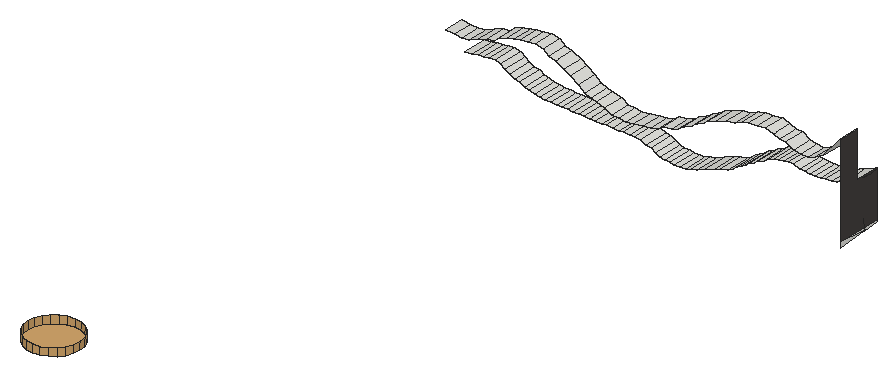
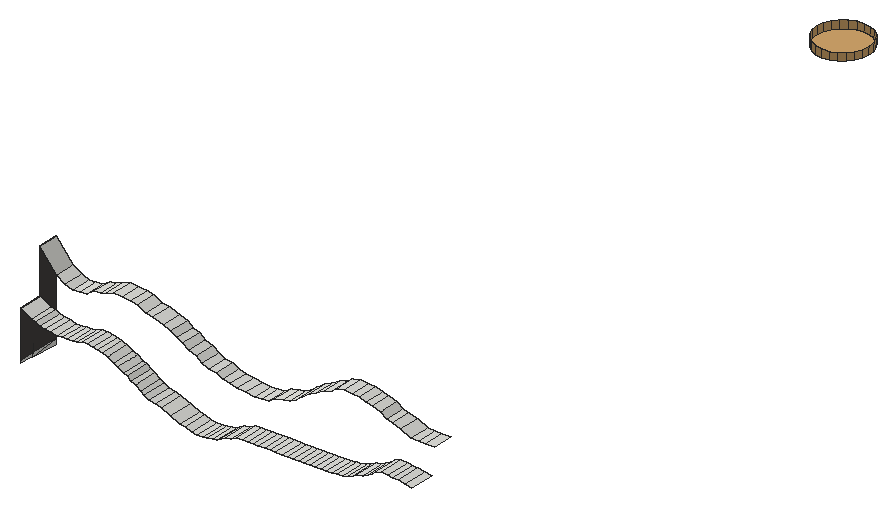
# SketchUp Ruby script. Lengths in inches.
U = 1.inch
M = Sketchup.active_model
def pt(a) = Geom::Point3d.new(a.map { |v| v * U })
def face(e, loops, mat)
  f = e.add_face(loops[0].map { |a| pt(a) })
  loops[1..].each { |l| e.add_face(l.map { |a| pt(a) }).erase! }
  f.material = f.back_material = mat if mat
  f
end
# faces: each face lists its corners as indices into pts; further lists are holes
def faces(e, pts, list, mat = nil) = list.each { |f| face(e, (f[0].is_a?(Array) ? f : [f]).map { |l| l.map { |i| pts[i] } }, mat) }
# xy, xz, yz: faces in a plane at the given z, y or x. An outline is a flat list of corners, or four numbers for a rectangle; further outlines are holes
def ring(l) = l.size == 4 ? [[l[0], l[1]], [l[2], l[1]], [l[2], l[3]], [l[0], l[3]]] : l.each_slice(2).to_a
def flat(e, list, mat, &to3) = list.each { |f| face(e, (f[0].is_a?(Array) ? f : [f]).map { |l| ring(l).map { |u, v| to3.(u, v) } }, mat) }
def xy(e, z, list, mat = nil) = flat(e, list, mat) { |x, y| [x, y, z] }
def xz(e, y, list, mat = nil) = flat(e, list, mat) { |x, z| [x, y, z] }
def yz(e, x, list, mat = nil) = flat(e, list, mat) { |y, z| [x, y, z] }
def lines(e, pts, list) = list.each { |a, b| e.add_line(pt(pts[a]), pt(pts[b])) }
# prism: a flat outline (further loops are holes) pulled along v
def prism(e, loops, v, mat = nil)
  f = face(e, loops, mat); d = Geom::Vector3d.new(v.map { |x| x * U })
  f.pushpull(f.normal.samedirection?(d) ? d.length : -d.length)
end
def box(e, o, s, mat = nil) = prism(e, [[o, [o[0] + s[0], o[1], o[2]], [o[0] + s[0], o[1] + s[1], o[2]], [o[0], o[1] + s[1], o[2]]]], [0, 0, s[2]], mat)
def at(x, y, z, deg = 0) = Geom::Transformation.translation(pt([x, y, z])) * Geom::Transformation.rotation(ORIGIN, Z_AXIS, deg.degrees)
def axes(o, x, y, z) = Geom::Transformation.new([*x, 0, *y, 0, *z, 0, *pt(o).to_a, 1])
def part(name) = M.definitions.add(name)
# library, detail: a bought-in or finely detailed component or shape, given as its bounding box
def library(name, o, s) = part(name).tap { |d| box(d.entities, o, s) }
def detail(e, o, s) = box(e.add_group.entities, o, s)
def put(e, d, t, mat = nil) = e.add_instance(d, t).tap { |i| i.material = mat if mat }
def group(e, t, mat = nil) = e.add_group.tap { |g| g.transformation = t; g.material = mat if mat }.entities
root = M.entities
M.materials.add("[Field Square Tile]").color = [211, 167, 108]
M.materials.add("[Granite Tile]1").color = [68, 65, 63]
xy(root,250.6875,[[1255.793,492.582,1255.081,492.675,1254.418,492.95,1253.848,493.387,1253.411,493.957,1253.136,494.62,1253.043,495.332,1253.136,496.043,1253.411,496.707,1253.848,497.276,1254.418,497.713,1255.081,497.988,1255.793,498.082,1256.504,497.988,1257.168,497.713,1257.737,497.276,1258.174,496.707,1258.449,496.043,1258.543,495.332,1258.449,494.62,1258.174,493.957,1257.737,493.387,1257.168,492.95,1256.504,492.675]],"[Field Square Tile]")
yz(root,1285.595,[[561.053,240.932,561.053,241.519,564.151,241.17],[564.185,241.167,564.151,241.17,564.184,241.173],[564.151,241.17,561.053,241.519,564.144,241.519,564.184,241.173],[564.184,241.173,564.144,241.519,565.74,241.519,565.74,241.293]])
yz(root,1285.595,[[561.053,241.519,561.053,251.165,563.178,251.165,563.178,246.426,565.74,246.426,565.74,241.519]],"[Granite Tile]1")
p = [[1266.017,563.178,241.17],[1266.017,565.74,241.17],[1266.487,565.74,241.121],[1266.487,563.178,241.121],[1267.093,565.74,241.09],[1267.093,563.178,241.09],
  [1267.66,565.74,241.138],[1267.66,563.178,241.138],[1268.3,565.74,241.346],[1268.3,563.178,241.346],[1265.019,563.178,241.332],[1265.019,565.74,241.332],
  [1265.487,565.74,241.243],[1265.487,563.178,241.243],[1264.6,563.178,241.566],[1264.6,565.74,241.566],[1268.891,565.74,241.456],[1268.891,563.178,241.456],
  [1269.826,565.74,241.847],[1269.826,563.178,241.847],[1264.094,563.178,241.837],[1264.094,565.74,241.837],[1263.521,563.178,241.967],[1263.521,565.74,241.967],
  [1270.831,565.74,242.229],[1270.831,563.178,242.229],[1262.94,563.178,242.199],[1262.94,565.74,242.199],[1262.314,563.178,242.277],[1262.314,565.74,242.277],
  [1271.392,565.74,242.424],[1271.392,563.178,242.424],[1256.467,563.178,242.35],[1256.467,565.74,242.35],[1257.049,565.74,242.342],[1257.049,563.178,242.342],
  [1257.631,565.74,242.334],[1257.631,563.178,242.334],[1258.213,565.74,242.326],[1258.213,563.178,242.326],[1258.933,565.74,242.317],[1258.933,563.178,242.317],
  [1259.403,565.74,242.312],[1259.403,563.178,242.312],[1260.044,565.74,242.304],[1260.044,563.178,242.304],[1260.708,565.74,242.296],[1260.708,563.178,242.296],
  [1261.16,565.74,242.291],[1261.16,563.178,242.291],[1261.798,565.74,242.283],[1261.798,563.178,242.283],[1252.985,563.178,242.466],[1252.985,565.74,242.466],
  [1253.561,565.74,242.428],[1253.561,563.178,242.428],[1254.14,565.74,242.403],[1254.14,563.178,242.403],[1254.72,565.74,242.385],[1254.72,563.178,242.385],
  [1255.302,565.74,242.371],[1255.302,563.178,242.371],[1255.884,565.74,242.36],[1255.884,563.178,242.36],[1272.11,565.74,242.605],[1272.11,563.178,242.605],
  [1251.857,563.178,242.599],[1251.857,565.74,242.599],[1252.417,565.74,242.518],[1252.417,563.178,242.518],[1251.304,563.178,242.75],[1251.304,565.74,242.75],
  [1272.623,565.74,242.907],[1272.623,563.178,242.907],[1250.816,563.178,242.921],[1250.816,565.74,242.921],[1250.325,563.178,243.216],[1250.325,565.74,243.216],
  [1272.995,565.74,243.144],[1272.995,563.178,243.144],[1273.544,565.74,243.516],[1273.544,563.178,243.516],[1249.777,563.178,243.332],[1249.777,565.74,243.332],
  [1249.232,563.178,243.589],[1249.232,565.74,243.589],[1274.018,565.74,243.711],[1274.018,563.178,243.711],[1248.751,563.178,243.88],[1248.751,565.74,243.88],
  [1274.349,565.74,244.02],[1274.349,563.178,244.02],[1248.374,563.178,244.194],[1248.374,565.74,244.194],[1244.586,563.178,243.992],[1244.586,565.74,243.992],
  [1245.289,565.74,244.076],[1245.289,563.178,244.076],[1274.793,565.74,244.206],[1274.793,563.178,244.206],[1245.988,565.74,244.207],[1245.988,563.178,244.207],
  [1246.573,565.74,244.266],[1246.573,563.178,244.266],[1247.777,563.178,244.387],[1247.777,565.74,244.387],[1275.382,565.74,244.569],[1275.382,563.178,244.569],
  [1247.114,565.74,244.296],[1247.114,563.178,244.296],[1275.852,565.74,244.757],[1275.852,563.178,244.757],[1276.469,565.74,245.125],[1276.469,563.178,245.125],
  [1261.665,561.053,245.064],[1261.665,563.178,245.064],[1262.375,563.178,244.949],[1262.375,561.053,244.949],[1263.089,563.178,244.867],[1263.089,561.053,244.867],
  [1263.995,563.178,245.007],[1263.995,561.053,245.007],[1264.939,563.178,245.121],[1264.939,561.053,245.121],[1260.952,561.053,245.459],[1260.952,563.178,245.459],
  [1265.704,563.178,245.254],[1265.704,561.053,245.254],[1276.973,565.74,245.32],[1276.973,563.178,245.32],[1280.674,563.178,245.272],[1280.674,565.74,245.272],
  [1281.232,565.74,245.235],[1281.232,563.178,245.235],[1281.786,565.74,245.216],[1281.786,563.178,245.216],[1282.351,565.74,245.34],[1282.351,563.178,245.34],
  [1266.456,563.178,245.41],[1266.456,561.053,245.41],[1277.455,565.74,245.411],[1277.455,563.178,245.411],[1279.021,563.178,245.552],[1279.021,565.74,245.552],
  [1279.629,565.74,245.346],[1279.629,563.178,245.346],[1280.123,565.74,245.309],[1280.123,563.178,245.309],[1282.983,565.74,245.423],[1282.983,563.178,245.423],
  [1267.09,563.178,245.775],[1267.09,561.053,245.775],[1278.003,565.74,245.481],[1278.003,563.178,245.481],[1283.561,565.74,245.516],[1283.561,563.178,245.516],
  [1260.077,561.053,245.671],[1260.077,563.178,245.671],[1278.485,565.74,245.59],[1278.485,563.178,245.59],[1283.941,565.74,245.763],[1283.941,563.178,245.763],
  [1259.402,561.053,245.834],[1259.402,563.178,245.834],[1258.814,561.053,246.129],[1258.814,563.178,246.129],[1267.886,563.178,245.88],[1267.886,561.053,245.88],
  [1284.41,565.74,245.896],[1284.41,563.178,245.896],[1268.599,563.178,246.16],[1268.599,561.053,246.16],[1285.595,565.74,246.426],[1285.595,563.178,246.426],
  [1258.183,561.053,246.633],[1258.183,563.178,246.633],[1269.196,563.178,246.573],[1269.196,561.053,246.573],[1257.369,561.053,247.185],[1257.369,563.178,247.185],
  [1269.986,563.178,246.902],[1269.986,561.053,246.902],[1245.192,561.053,246.79],[1245.192,563.178,246.79],[1245.971,563.178,246.747],[1245.971,561.053,246.747],
  [1246.718,563.178,246.831],[1246.718,561.053,246.831],[1244.238,561.053,246.838],[1244.238,563.178,246.838],[1247.76,563.178,247.251],[1247.76,561.053,247.251],
  [1270.588,563.178,247.347],[1270.588,561.053,247.347],[1256.657,561.053,247.553],[1256.657,563.178,247.553],[1248.634,563.178,247.546],[1248.634,561.053,247.546],
  [1271.262,563.178,247.615],[1271.262,561.053,247.615],[1249.296,563.178,247.657],[1249.296,561.053,247.657],[1255.766,561.053,248.059],[1255.766,563.178,248.059],
  [1271.849,563.178,248.057],[1271.849,561.053,248.057],[1249.929,563.178,248.162],[1249.929,561.053,248.162],[1255.075,561.053,248.257],[1255.075,563.178,248.257],
  [1272.614,563.178,248.322],[1272.614,561.053,248.322],[1250.723,563.178,248.408],[1250.723,561.053,248.408],[1281.411,561.053,248.295],[1281.411,563.178,248.295],
  [1282.12,563.178,248.218],[1282.12,561.053,248.218],[1282.937,563.178,248.558],[1282.937,561.053,248.558],[1254.544,561.053,248.687],[1254.544,563.178,248.687],
  [1273.725,563.178,248.655],[1273.725,561.053,248.655],[1280.7,561.053,248.42],[1280.7,563.178,248.42],[1251.422,563.178,248.521],[1251.422,561.053,248.521],
  [1279.903,561.053,248.895],[1279.903,563.178,248.895],[1252.116,563.178,248.723],[1252.116,561.053,248.723],[1283.872,563.178,249.022],[1283.872,561.053,249.022],
  [1252.815,563.178,248.801],[1252.815,561.053,248.801],[1253.712,561.053,248.851],[1253.712,563.178,248.851],[1274.498,563.178,248.795],[1274.498,561.053,248.795],
  [1275.361,563.178,249.194],[1275.361,561.053,249.194],[1279.199,561.053,248.962],[1279.199,563.178,248.962],[1278.56,561.053,249.206],[1278.56,563.178,249.206],
  [1285.595,563.178,251.165],[1285.595,561.053,251.165],[1276.034,563.178,249.323],[1276.034,561.053,249.323],[1277.815,561.053,249.478],[1277.815,563.178,249.478],
  [1276.957,563.178,249.406],[1276.957,561.053,249.406],[1255.793,492.582,251.5],[1255.081,492.675,251.5],[1255.081,492.675,250.6875],[1255.793,492.582,250.6875],
  [1256.504,492.675,251.5],[1256.504,492.675,250.6875],[1254.418,492.95,251.5],[1254.418,492.95,250.6875],[1257.168,492.95,251.5],[1257.168,492.95,250.6875],
  [1253.848,493.387,251.5],[1253.848,493.387,250.6875],[1257.737,493.387,251.5],[1257.737,493.387,250.6875],[1253.411,493.957,251.5],[1253.411,493.957,250.6875],
  [1258.174,493.957,251.5],[1258.174,493.957,250.6875],[1253.136,494.62,251.5],[1253.136,494.62,250.6875],[1258.449,494.62,251.5],[1258.449,494.62,250.6875],
  [1253.043,495.332,251.5],[1253.043,495.332,250.6875],[1258.543,495.332,251.5],[1258.543,495.332,250.6875],[1253.136,496.043,251.5],[1253.136,496.043,250.6875],
  [1258.449,496.043,251.5],[1258.449,496.043,250.6875],[1253.411,496.707,251.5],[1253.411,496.707,250.6875],[1258.174,496.707,251.5],[1258.174,496.707,250.6875],
  [1253.848,497.276,251.5],[1253.848,497.276,250.6875],[1257.737,497.276,251.5],[1257.737,497.276,250.6875],[1254.418,497.713,251.5],[1254.418,497.713,250.6875],
  [1257.168,497.713,251.5],[1257.168,497.713,250.6875],[1255.081,497.988,251.5],[1255.081,497.988,250.6875],[1256.504,497.988,251.5],[1256.504,497.988,250.6875],
  [1255.793,498.082,251.5],[1255.793,498.082,250.6875],[1285.595,564.963,246.171],[1285.595,563.948,246.265],[1285.595,565.74,246.273],[1285.595,564.144,241.519],
  [1285.595,564.042,242.384]]
faces(root,p,[[0,1,2,3],[3,2,4,5],[5,4,6,7],[7,6,8,9],[10,11,12,13],[13,12,1,0],[14,15,11,10],[9,8,16,17],
  [17,16,18,19],[20,21,15,14],[22,23,21,20],[19,18,24,25],[26,27,23,22],[28,29,27,26],[25,24,30,31],[32,33,34,35],
  [35,34,36,37],[37,36,38,39],[39,38,40,41],[41,40,42,43],[43,42,44,45],[45,44,46,47],[47,46,48,49],[49,48,50,51],
  [51,50,29,28],[52,53,54,55],[55,54,56,57],[57,56,58,59],[59,58,60,61],[61,60,62,63],[63,62,33,32],[31,30,64,65],
  [66,67,68,69],[69,68,53,52],[70,71,67,66],[65,64,72,73],[74,75,71,70],[76,77,75,74],[73,72,78,79],[79,78,80,81],
  [82,83,77,76],[84,85,83,82],[81,80,86,87],[88,89,85,84],[87,86,90,91],[92,93,89,88],[94,95,96,97],[91,90,98,99],
  [97,96,100,101],[101,100,102,103],[104,105,93,92],[99,98,106,107],[103,102,108,109],[109,108,105,104],[107,106,110,111],[111,110,112,113],
  [114,115,116,117],[117,116,118,119],[119,118,120,121],[121,120,122,123],[124,125,115,114],[123,122,126,127],[113,112,128,129],[130,131,132,133],
  [133,132,134,135],[135,134,136,137],[127,126,138,139],[129,128,140,141],[142,143,144,145],[145,144,146,147],[147,146,131,130],[137,136,148,149],
  [139,138,150,151],[141,140,152,153],[149,148,154,155],[156,157,125,124],[153,152,158,159],[155,154,160,161],[159,158,143,142],[162,163,157,156],
  [164,165,163,162],[151,150,166,167],[161,160,168,169],[167,166,170,171],[169,168,172,173],[174,175,165,164],[171,170,176,177],[178,179,175,174],
  [177,176,180,181],[182,183,184,185],[185,184,186,187],[188,189,183,182],[187,186,190,191],[181,180,192,193],[194,195,179,178],[191,190,196,197],
  [193,192,198,199],[197,196,200,201],[202,203,195,194],[199,198,204,205],[201,200,206,207],[208,209,203,202],[205,204,210,211],[207,206,212,213],
  [214,215,216,217],[217,216,218,219],[220,221,209,208],[211,210,222,223],[224,225,215,214],[213,212,226,227],[228,229,225,224],[227,226,230,231],
  [219,218,232,233],[231,230,234,235],[236,237,221,220],[223,222,238,239],[235,234,237,236],[239,238,240,241],[242,243,229,228],[244,245,243,242],
  [233,232,246,247],[241,240,248,249],[250,251,245,244],[249,248,252,253],[253,252,251,250]])
faces(root,p,[[254,255,256,257],[258,254,257,259],[255,260,261,256],[262,258,259,263],[260,264,265,261],[266,262,263,267],[264,268,269,265],[270,266,267,271],
  [268,272,273,269],[274,270,271,275],[272,276,277,273],[278,274,275,279],[276,280,281,277],[282,278,279,283],[280,284,285,281],[286,282,283,287],
  [284,288,289,285],[290,286,287,291],[288,292,293,289],[294,290,291,295],[292,296,297,293],[298,294,295,299],[296,300,301,297],[300,298,299,301]],"[Field Square Tile]")
lines(root,p,[[302,303],[304,302],[305,306]])
